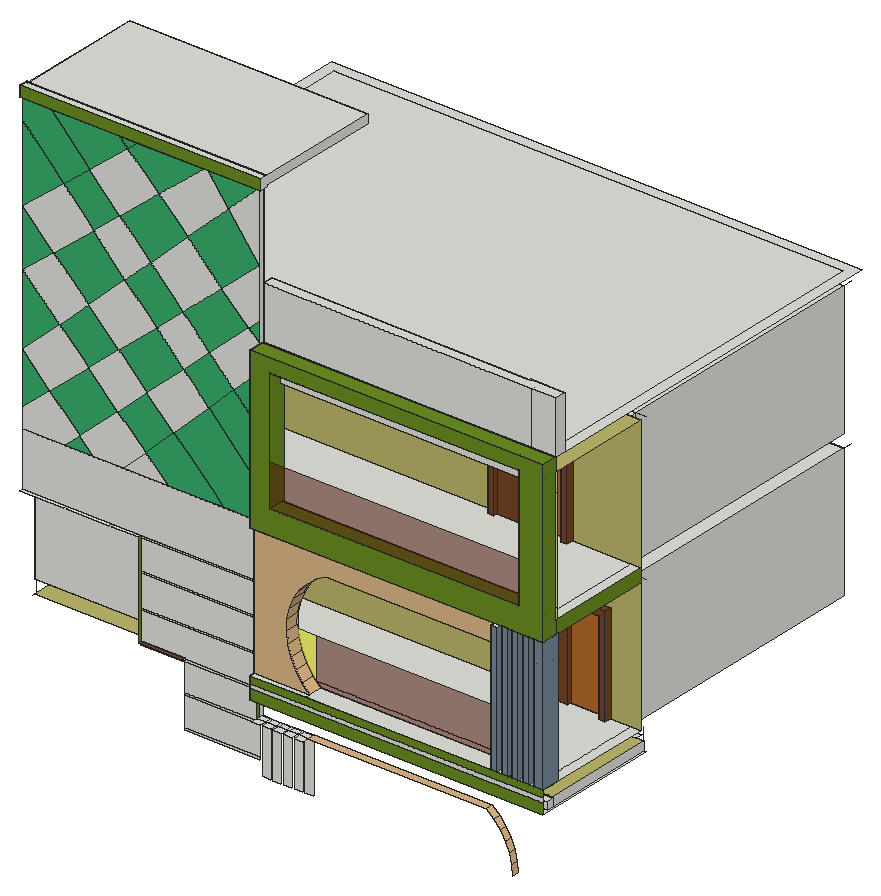
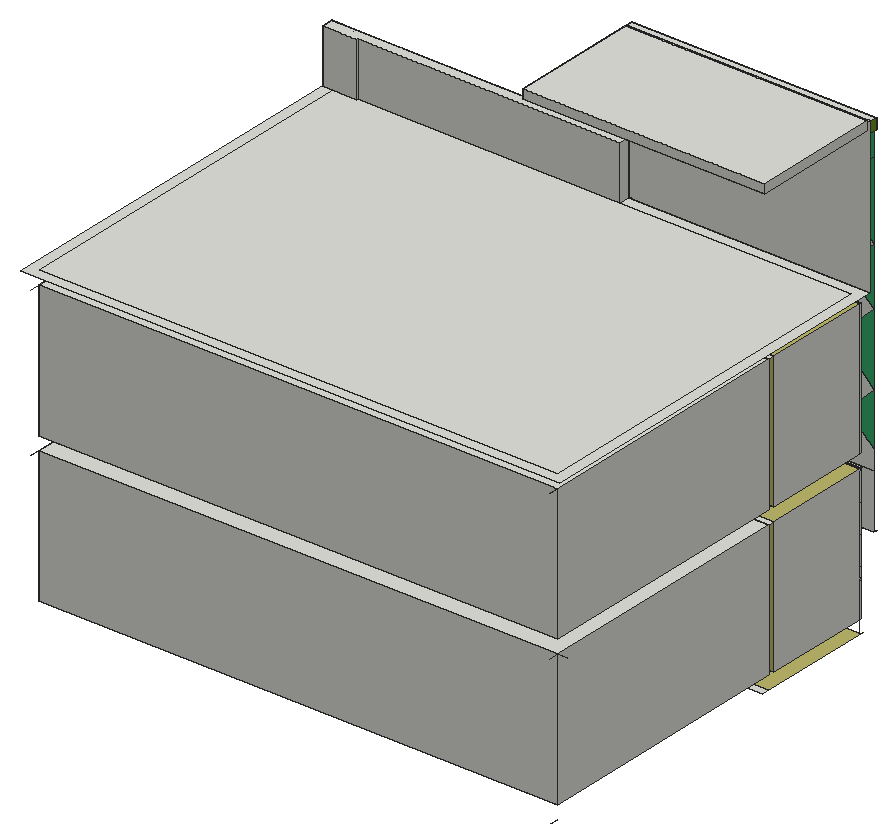
# SketchUp Ruby script. Lengths in inches.
U = 1.inch
M = Sketchup.active_model
def pt(a) = Geom::Point3d.new(a.map { |v| v * U })
def face(e, loops, mat)
  f = e.add_face(loops[0].map { |a| pt(a) })
  loops[1..].each { |l| e.add_face(l.map { |a| pt(a) }).erase! }
  f.material = f.back_material = mat if mat
  f
end
# faces: each face lists its corners as indices into pts; further lists are holes
def faces(e, pts, list, mat = nil) = list.each { |f| face(e, (f[0].is_a?(Array) ? f : [f]).map { |l| l.map { |i| pts[i] } }, mat) }
# xy, xz, yz: faces in a plane at the given z, y or x. An outline is a flat list of corners, or four numbers for a rectangle; further outlines are holes
def ring(l) = l.size == 4 ? [[l[0], l[1]], [l[2], l[1]], [l[2], l[3]], [l[0], l[3]]] : l.each_slice(2).to_a
def flat(e, list, mat, &to3) = list.each { |f| face(e, (f[0].is_a?(Array) ? f : [f]).map { |l| ring(l).map { |u, v| to3.(u, v) } }, mat) }
def xy(e, z, list, mat = nil) = flat(e, list, mat) { |x, y| [x, y, z] }
def xz(e, y, list, mat = nil) = flat(e, list, mat) { |x, z| [x, y, z] }
def yz(e, x, list, mat = nil) = flat(e, list, mat) { |y, z| [x, y, z] }
def lines(e, pts, list) = list.each { |a, b| e.add_line(pt(pts[a]), pt(pts[b])) }
# prism: a flat outline (further loops are holes) pulled along v
def prism(e, loops, v, mat = nil)
  f = face(e, loops, mat); d = Geom::Vector3d.new(v.map { |x| x * U })
  f.pushpull(f.normal.samedirection?(d) ? d.length : -d.length)
end
def box(e, o, s, mat = nil) = prism(e, [[o, [o[0] + s[0], o[1], o[2]], [o[0] + s[0], o[1] + s[1], o[2]], [o[0], o[1] + s[1], o[2]]]], [0, 0, s[2]], mat)
def at(x, y, z, deg = 0) = Geom::Transformation.translation(pt([x, y, z])) * Geom::Transformation.rotation(ORIGIN, Z_AXIS, deg.degrees)
def axes(o, x, y, z) = Geom::Transformation.new([*x, 0, *y, 0, *z, 0, *pt(o).to_a, 1])
def part(name) = M.definitions.add(name)
# library, detail: a bought-in or finely detailed component or shape, given as its bounding box
def library(name, o, s) = part(name).tap { |d| box(d.entities, o, s) }
def detail(e, o, s) = box(e.add_group.entities, o, s)
def put(e, d, t, mat = nil) = e.add_instance(d, t).tap { |i| i.material = mat if mat }
def group(e, t, mat = nil) = e.add_group.tap { |g| g.transformation = t; g.material = mat if mat }.entities
root = M.entities
M.materials.add("[0036_BurlyWood]").color = [222, 184, 135]
M.materials.add("[0057_DarkKhaki]").color = [189, 183, 107]
M.materials.add("[0061_OliveDrab]").color = [107, 142, 35]
M.materials.add("[0074_SeaGreen]").color = [57, 173, 108]
M.materials.add("[0110_LightSlateGray]").color = [119, 136, 153]
M.materials.add("[Sandstone]").color = [118, 81, 52]
M.materials.add("[Translucent Glass Dark Green]").color = [91, 24, 11]
M.materials["[Translucent Glass Dark Green]"].alpha = 0.5
M.materials.add("[Translucent Glass Gold]").color = [255, 254, 26]
M.materials["[Translucent Glass Gold]"].alpha = 0.6
M.materials.add("[Translucent Glass Gray]").color = [128, 128, 128]
M.materials["[Translucent Glass Gray]"].alpha = 0.5
M.materials.add("[Wood Bamboo]").color = [177, 105, 43]
M.materials.add("[Wood Cherry Original]").color = [152, 86, 42]
M.materials.add("[Wood Veneer 01]").color = [120, 70, 37]
xy(root,302.01,[[383.79,177.4375,383.79,179.4375,386.62,179.4375,386.62,178.4375,395.22,178.4375,395.22,179.4375,398.06,179.4375,398.06,177.4375]],"[Wood Veneer 01]")
xy(root,303.76,[[383.79,177.4375,398.06,177.4375,398.06,179.4375,395.22,179.4375,395.22,178.4375,386.62,178.4375,386.62,179.4375,383.79,179.4375]],"[Wood Veneer 01]")
xy(root,336,[[379.35,179.4375,409.35,182.4375]])
xy(root,336,[[379.35,176.4375,409.35,179.4375],[409.35,176.4375,439.35,182.4375]],"[Wood Veneer 01]")
xy(root,338.33,[[301.39,179.4375,326.48,182.4375],[329.2,179.4375,351.57,182.4375]],"[Wood Cherry Original]")
xy(root,341.33,[[298.39,179.4375,354.57,182.4375]],"[Wood Cherry Original]")
xy(root,342,[[373.35,176.4375,445.35,182.4375]],"[Wood Veneer 01]")
xy(root,345.55,[[214.69,67.75,222.11,73.75],[224.38,67.75,231.79,73.75],[234.07,67.75,241.48,73.75],[243.75,67.75,251.17,73.75],[253.44,67.75,260.86,73.75],
  [214.69,73.75,222.11,79.75],[222.11,73.75,224.38,79.75],[224.38,73.75,231.79,79.75],[231.79,73.75,234.07,79.75],[234.07,73.75,241.48,79.75],
  [241.48,73.75,243.75,79.75],[243.75,73.75,251.17,79.75],[251.17,73.75,253.44,79.75],[253.44,73.75,260.86,79.75]])
xy(root,345.55,[[260.86,73.75,422.69,79.75]],"[0036_BurlyWood]")
xy(root,363.8125,[[214.69,65.75,214.69,73.75,477.8125,73.75,477.8125,182.4375,480,182.4375,480,65.75]])
xy(root,369.44,[[107.35,73.75,146.78,76.75]],"[Sandstone]")
xy(root,370.625,[[214.69,73.75,477.8125,79.75,477.8125,73.75]])
xy(root,372,[[9,182.4375,471,188.4375]])
xy(root,372,[[9,79.75,477.8125,182.4375]],"[0057_DarkKhaki]")
xy(root,384,[[214.69,65.75,264.77,70.3125],[264.77,65.75,432.6,82.75],[432.6,65.75,438.3,82.75],[438.3,65.75,442.22,82.75],[442.22,65.75,447.93,82.75],
  [447.93,65.75,451.85,82.75],[451.85,65.75,457.55,82.75],[457.55,65.75,461.47,82.75],[461.47,65.75,467.18,82.75],[467.18,65.75,471.78,82.75],
  [471.78,65.75,480,76.75],[214.69,70.3125,264.77,76.75],[214.69,76.75,264.77,79.75],[471.78,76.75,480,77.8125],[471.78,77.8125,480,82.75],
  [9,79.75,214.69,81.3125],[214.69,79.75,264.77,79.75,264.77,82.75,244.77,82.75,244.77,82.4375,214.69,82.4375],[9,81.3125,214.69,81.3125,214.69,82.75,480,82.75,480,176.4375,471,176.4375,471,88.75,9,88.75],[214.69,82.4375,244.77,82.75],[9,88.75,471,88.75,471,176.4375,452.43,176.4375,452.43,170.4375,446.43,170.4375,446.43,176.4375,416.43,176.4375,416.43,173.4375,386.43,173.4375,386.43,170.4375,380.43,170.4375,380.43,176.4375,9,176.4375],
  [380.43,170.4375,386.43,176.4375],[446.43,170.4375,452.43,176.4375],[386.43,173.4375,416.43,176.4375],[9,182.4375,471,417.3125]])
xy(root,415.43,[[290.01,173.4375,348.2,176.4375]])
xy(root,418.43,[[293.01,173.4375,319.1,176.4375],[322.56,173.4375,345.2,176.4375]],"[Wood Cherry Original]")
xy(root,433.625,[[389.68,170.4375,390.18,171.4375],[389.68,171.4375,390.18,173.4375]],"[Wood Veneer 01]")
xy(root,434.43,[[389.68,171.4375,390.18,173.4375]],"[Wood Veneer 01]")
xy(root,440.6875,[[389.68,171.4375,390.18,173.4375]],"[Wood Veneer 01]")
xy(root,441.5,[[389.68,170.4375,390.18,171.4375],[389.68,171.4375,390.18,173.4375]],"[Wood Veneer 01]")
xy(root,455,[[0,73.75,39.7,76.75],[42.34,73.75,80.57,76.75],[83.22,73.75,107.35,76.75]])
xy(root,468,[[386.43,173.4375,416.43,176.4375]])
xy(root,468,[[386.43,170.4375,416.43,173.4375],[416.43,170.4375,446.43,176.4375]],"[Wood Veneer 01]")
xy(root,474,[[380.43,170.4375,452.43,176.4375]],"[Wood Veneer 01]")
xy(root,478.24,[[293.01,173.4375,319.1,176.4375],[322.56,173.4375,345.2,176.4375]],"[Wood Cherry Original]")
xy(root,481.24,[[290.01,173.4375,348.2,176.4375]])
xy(root,484.84,[[279.79,82.4375,471.78,82.75]])
xy(root,484.84,[[279.79,70.3125,471.78,76.75]],"[0036_BurlyWood]")
xy(root,501.3125,[[432.6,65.75,438.3,82.75]])
xy(root,504,[[214.69,65.75,442.22,67.21],[442.22,65.75,447.93,70.3125],[447.93,65.75,451.85,67.21],[451.85,65.75,457.55,67.21],[457.55,65.75,461.47,67.21],
  [461.47,65.75,467.18,67.21],[467.18,65.75,471.78,67.21],[471.78,65.75,473.53,67.21],[473.53,65.75,480,67.21],[214.69,67.21,442.22,70.3125],
  [447.93,67.21,451.85,70.3125],[451.85,67.21,457.55,70.3125],[457.55,67.21,461.47,70.3125],[461.47,67.21,467.18,70.3125],[467.18,67.21,471.78,70.3125],
  [471.78,67.21,473.53,70.3125],[473.53,67.21,480,76.75],[214.69,70.3125,442.22,76.75],[442.22,70.3125,447.93,76.75],[447.93,70.3125,451.85,76.75],
  [451.85,70.3125,457.55,76.75],[457.55,70.3125,461.47,76.75],[461.47,70.3125,467.18,76.75],[467.18,70.3125,471.78,76.75],[471.78,70.3125,473.53,76.75],
  [9,76.75,214.69,79.75],[214.69,76.75,442.22,79.75],[442.22,76.75,447.93,79.75],[447.93,76.75,451.85,79.75],[451.85,76.75,457.55,79.75],
  [457.55,76.75,461.47,79.75],[461.47,76.75,467.18,79.75],[467.18,76.75,471.78,79.75],[471.78,76.75,473.53,79.75],[473.53,76.75,480,79.75],
  [9,79.75,214.69,81.3125],[214.69,79.75,451.85,82.4375],[451.85,79.75,457.55,82.4375],[457.55,79.75,461.47,82.4375],[461.47,79.75,467.18,82.4375],
  [467.18,79.75,471.78,82.4375],[471.78,79.75,480,82.75],[214.69,82.4375,451.85,82.75],[451.85,82.4375,457.55,82.75],[457.55,82.4375,461.47,82.75],
  [461.47,82.4375,467.18,82.75],[467.18,82.4375,471.78,82.75],[9,176.4375,471,182.4375],[9,182.4375,471,417.3125]])
xy(root,504,[[9,81.3125,9,176.4375,480,176.4375,480,82.75,214.69,82.75,214.69,81.3125]],"[0057_DarkKhaki]")
xy(root,504.25,[[442.22,65.75,447.93,67.21],[442.22,67.21,447.93,79.75],[442.22,79.75,447.93,82.75]])
xy(root,516,[[232.86,79.75,471,79.75,471,176.4375,418.0625,176.4375,418.0625,170.4375,412.0625,170.4375,412.0625,176.4375,382.0625,176.4375,382.0625,173.4375,352.0625,173.4375,352.0625,170.4375,346.0625,170.4375,346.0625,176.4375,9,176.4375,9,81.3125,214.69,81.3125,214.69,81.21,232.86,81.21],[9,79.75,214.69,81.3125],[214.69,79.75,232.86,81.21],[471,79.75,480,176.4375],[346.0625,170.4375,352.0625,176.4375],
  [412.0625,170.4375,418.0625,176.4375],[352.0625,173.4375,382.0625,176.4375],[9,182.4375,471,417.3125]])
xy(root,525.77,[[232.86,65.75,458.23,79.75]],"[0061_OliveDrab]")
xy(root,557.24,[[255.7,173.4375,311.2,176.4375]])
xy(root,560.24,[[258.7,173.4375,283.45,176.4375],[285.78,173.4375,308.2,176.4375]],"[Wood Cherry Original]")
xy(root,560.85,[[354.3,171.4375,355.24,173.4375]])
xy(root,563.35,[[354.3,172.4375,355.24,173.4375]],"[Wood Veneer 01]")
xy(root,570.73,[[354.3,172.4375,355.24,173.4375]])
xy(root,573.23,[[354.3,171.4375,355.24,173.4375]],"[Wood Veneer 01]")
xy(root,600,[[352.0625,170.4375,382.0625,173.4375],[382.0625,170.4375,412.0625,176.4375]],"[Wood Veneer 01]")
xy(root,606,[[346.0625,170.4375,418.0625,176.4375]],"[Wood Veneer 01]")
xy(root,609.74,[[258.7,173.4375,283.45,176.4375],[285.78,173.4375,308.2,176.4375]],"[Wood Cherry Original]")
xy(root,612.74,[[255.7,173.4375,311.2,176.4375]],"[Wood Cherry Original]")
xy(root,622.99,[[458.2,75.25,232.83,76.58,232.86,81.21,458.23,79.88,458.23,79.75]])
xy(root,636,[[458.2,75.25,232.86,76.58,232.86,79.75,458.23,79.75],[232.83,76.58,232.86,76.58,232.86,79.75,232.85,79.75],[9,79.75,214.69,81.3125],[214.69,79.75,232.85,79.75,232.86,81.21,214.69,81.21],[232.86,79.75,232.86,81.21,214.69,81.21,214.69,81.3125,232.86,81.21,458.23,79.88,458.23,79.75],
  [232.85,79.75,232.86,79.75,232.86,81.21],[9,176.4375,471,182.4375],[9,182.4375,471,417.3125]])
xy(root,636,[[480,79.75,458.23,79.88,232.86,81.21,214.69,81.3125,9,81.3125,9,176.4375,480,176.4375]],"[0057_DarkKhaki]")
xy(root,636,[[232.86,65.75,458.23,67.21],[232.86,67.21,232.86,76.58,458.2,75.25,458.23,79.75,458.23,67.21]],"[0061_OliveDrab]")
xy(root,648,[[214.69,79.75,458.23,79.75,458.23,79.88,214.69,81.3125],[458.23,79.75,480,79.75,458.23,79.88],[480,79.75,480,79.88,458.23,79.88],[458.23,79.88,214.69,81.3125,214.72,90.3125,449.23,88.93,449.23,90.21,480,90.21,480,82.71,458.23,82.71],[458.23,79.88,480,80.14],
  [458.23,80.14,480,81.21],[458.23,81.21,480,82.71],[0,81.3125,214.69,81.3125,214.72,90.3125,9,90.3125,9,417.3125,471,417.3125,471,90.21,480,90.21,480,426.3125,0,426.3125],[449.23,88.93,449.23,90.21,471,90.21,471,417.3125,9,417.3125,9,90.3125,214.72,90.3125]])
xy(root,648,[[214.69,65.75,480,79.75]],"[0061_OliveDrab]")
xy(root,696,[[458.23,79.88,480,79.88,480,90.21,449.23,90.21,449.23,88.93,214.72,90.3125,214.69,81.3125]])
xy(root,774.38,[[0,76.75,22.45,79.75],[22.45,76.75,85.57,79.75],[85.57,76.75,107.35,79.75],[107.35,76.75,166.47,79.75],[166.47,76.75,214.69,79.75]])
xy(root,774.38,[[0,73.75,22.45,76.75],[22.45,73.75,85.57,76.75],[85.57,73.75,107.35,76.75],[107.35,73.75,166.47,76.75],[166.47,73.75,166.47,76.75,214.69,76.75,214.69,81.3125,217.75,81.3125,217.75,73.75]],"[0061_OliveDrab]")
xy(root,775.875,[[2.13,81.3125,217.75,194.875]])
xy(root,784.0625,[[0,73.75,217.75,79.75],[0,79.75,2.13,81.3125],[2.13,79.75,217.75,81.3125],[2.13,81.3125,217.75,194.875]])
xz(root,65.75,[[214.69,373.91,480,377.57],[442.22,504,447.93,504.25]])
xz(root,65.75,[[214.69,363.8125,480,373.91],[214.69,377.57,480,384],[[214.69,504,442.22,504,442.22,504.25,447.93,504.25,447.93,504,480,504,480,648,214.69,648],[232.86,525.77,458.23,636]]],"[0061_OliveDrab]")
xz(root,65.75,[[432.6,384,438.3,501.3125],[442.22,384,447.93,504],[451.85,384,457.55,504],[461.47,384,467.18,504],[471.78,384,480,504]],"[0110_LightSlateGray]")
xz(root,65.75,[[232.86,525.77,458.23,563.72]],"[Translucent Glass Dark Green]")
xz(root,70.3125,[[471.78,484.84,473.53,504]])
xz(root,70.3125,[[214.69,384,264.77,384,257.77,391.25,252.07,399.57,247.82,408.71,245.15,418.43,244.12,428.46,244.77,438.52,247.08,448.33,250.99,457.625,256.375,466.14,263.1,473.65,270.98,479.94,279.79,484.84,471.78,484.84,471.78,504,214.69,504]],"[0036_BurlyWood]")
xz(root,73.75,[[214.69,363.8125,477.8125,370.625]])
xz(root,73.75,[[0,774.38,217.75,784.0625]],"[0061_OliveDrab]")
xz(root,76.75,[[146.78,310.89,214.69,312.74],[146.78,312.74,214.69,339.34],[146.78,339.34,214.69,341.2],[146.78,341.2,214.69,341.2,214.69,366.59,107.35,366.59,107.35,369.44,146.78,369.44],[107.35,366.59,146.78,368.45],
  [146.78,366.59,214.69,368.45],[107.35,368.45,146.78,369.44],[146.78,368.45,214.69,368.45,214.69,394.84,107.35,394.84,107.35,369.44,146.78,369.44],[107.35,394.84,214.69,396.7],[107.35,396.7,214.69,424.34],
  [107.35,424.34,214.69,426.2],[107.35,426.2,214.69,453.13],[107.35,453.13,214.69,455],[0,455,214.69,504],[0,504,38.29,504,52.01,516.65,24.94,543.56,0,521.52],
  [64.73,504,91.18,504,111.25,523.71,86.25,548.21,52.01,516.65],[91.18,504,131.37,504,111.25,523.71],[24.94,543.56,59.68,574.24,33.18,600.2,0,568.36],[86.25,548.21,112.7,572.59,86.87,598.27,59.68,574.24],[136.72,548.71,168.17,579.59,145.625,602.94,112.7,572.59],
  [86.87,598.27,121.02,628.4375,92.93,657.54,59.51,625.47],[33.18,600.2,59.51,625.47,28.14,656.66,0,632.72],[191.26,602.27,214.69,625.27,214.69,647.875,204.84,657.53,169.24,624.71],[145.625,602.94,169.24,624.71,144.9,649.53,121.02,628.4375],[144.9,649.53,180.71,681.17,149.46,711.79,115.66,679.35],
  [28.14,656.66,64.18,687.33,36.96,715.53,0,684.63],[204.84,657.53,214.69,666.6,214.69,711.19,180.71,681.17],[92.93,657.54,115.66,679.35,87.97,707.58,64.18,687.33],[87.97,707.58,123.18,737.54,95.6,764.5625,60.7,735.38],[214.69,711.19,214.69,774.38,186.85,747.67],
  [149.46,711.79,186.85,747.67,166.47,774.38,123.18,737.54]])
xz(root,76.75,[[38.29,504,64.73,504,52.01,516.65],[131.37,504,181.6875,504,136.72,548.71,111.25,523.71],[181.6875,504,214.69,504,214.69,531.38,168.17,579.59,136.72,548.71],[52.01,516.65,86.25,548.21,59.68,574.24,24.94,543.56],[0,521.52,24.94,543.56,0,568.36],
  [111.25,523.71,136.72,548.71,112.7,572.59,86.25,548.21],[214.69,531.38,214.69,578.38,191.26,602.27,168.17,579.59],[0,568.36,33.18,600.2,0,632.72],[112.7,572.59,145.625,602.94,121.02,628.4375,86.87,598.27],[59.68,574.24,86.87,598.27,59.51,625.47,33.18,600.2],
  [214.69,578.38,214.69,625.27,191.26,602.27],[168.17,579.59,191.26,602.27,169.24,624.71,145.625,602.94],[169.24,624.71,204.84,657.53,180.71,681.17,144.9,649.53],[59.51,625.47,92.93,657.54,64.18,687.33,28.14,656.66],[121.02,628.4375,144.9,649.53,115.66,679.35,92.93,657.54],
  [0,632.72,28.14,656.66,0,684.63],[214.69,647.875,214.69,666.6,204.84,657.53],[115.66,679.35,149.46,711.79,123.18,737.54,87.97,707.58],[180.71,681.17,214.69,711.19,186.85,747.67,149.46,711.79],[0,684.63,36.96,715.53,0,753.83],
  [64.18,687.33,87.97,707.58,60.7,735.38,36.96,715.53],[36.96,715.53,60.7,735.38,22.45,774.38,0,774.38,0,753.83],[60.7,735.38,95.6,764.5625,85.57,774.38,22.45,774.38],[123.18,737.54,166.47,774.38,107.35,774.38,95.6,764.5625],[186.85,747.67,214.69,774.38,166.47,774.38],
  [95.6,764.5625,107.35,774.38,85.57,774.38]],"[0074_SeaGreen]")
xz(root,79.75,[[214.69,296.15,222.11,345.55],[224.38,296.15,231.79,345.55],[234.07,296.15,241.48,345.55],[243.75,296.15,251.17,345.55],[253.44,296.15,260.86,345.55],
  [214.69,370.625,477.8125,372],[9,384,214.69,504],[214.69,504,214.69,516,480,516,480,504,447.93,504,447.93,504.25,442.22,504.25,442.22,504],[442.22,504,447.93,504.25],[9,516,214.69,636],
  [232.86,516,232.86,525.77,458.23,525.77,458.23,636,214.69,636,214.69,648,480,648,480,516]])
xz(root,79.88,[[458.23,648,480,696]])
xz(root,81.21,[[214.69,516,232.86,636]])
xz(root,81.3125,[[0,647.875,214.69,648],[0,648,0,784.0625,2.13,784.0625,2.13,775.875,217.75,775.875,217.75,774.38,214.69,774.38,214.69,648]])
xz(root,82.4375,[[214.69,384,244.77,384,244.77,422.09,244.44,425.34,244.12,428.46,244.77,438.52,247.08,448.33,250.99,457.625,256.375,466.14,263.1,473.65,270.98,479.94,279.79,484.84,471.78,484.84,471.78,504,214.69,504]],"[0057_DarkKhaki]")
xz(root,82.75,[[214.69,384,214.69,504,442.22,504,442.22,484.84,438.3,484.84,438.3,501.3125,432.6,501.3125,432.6,484.84,279.79,484.84,270.98,479.94,263.1,473.65,256.375,466.14,250.99,457.625,247.08,448.33,244.77,438.52,244.12,428.46,244.44,425.34,244.77,422.09,244.77,384],[244.77,384,244.77,422.09,245.15,418.43,247.82,408.71,252.07,399.57,257.77,391.25,264.77,384],[432.6,384,438.3,425.34],[438.3,384,442.22,425.34],[442.22,384,447.93,425.34],
  [447.93,384,451.85,425.34],[451.85,384,457.55,425.34],[457.55,384,461.47,425.34],[461.47,384,467.18,425.34],[467.18,384,471.78,425.34],
  [471.78,384,480,504],[244.77,422.09,244.44,425.34,244.77,425.34],[244.44,425.34,244.12,428.46,244.77,438.52,244.77,425.34],[432.6,425.34,438.3,484.84],[442.22,425.34,447.93,484.84],
  [451.85,425.34,457.55,484.84],[461.47,425.34,467.18,484.84],[432.6,484.84,438.3,501.3125],[442.22,484.84,447.93,504],[447.93,484.84,451.85,504],
  [451.85,484.84,457.55,504],[457.55,484.84,461.47,504],[461.47,484.84,467.18,504],[467.18,484.84,471.78,504],[442.22,504,447.93,504.25]])
xz(root,82.75,[[264.77,384,432.6,384,432.6,425.34,261.27,425.34,261.27,387.625]],"[Translucent Glass Dark Green]")
xz(root,82.75,[[261.27,387.625,257.77,391.25,252.07,399.57,247.82,408.71,245.15,418.43,244.77,422.09,244.77,425.34,261.27,425.34]],"[Translucent Glass Gold]")
xz(root,90.21,[[449.23,648,480,696]])
xz(root,170.4375,[[380.43,384,386.43,384,386.43,468,446.43,468,446.43,384,452.43,384,452.43,474,380.43,474],[389.68,433.625,390.18,441.5],[346.0625,516,352.0625,516,352.0625,600,412.0625,600,412.0625,516,418.0625,516,418.0625,606,346.0625,606]],"[Wood Veneer 01]")
xz(root,171.4375,[[389.68,434.43,390.18,440.6875]])
xz(root,171.4375,[[354.3,560.85,355.24,573.23]],"[Wood Veneer 01]")
xz(root,172.4375,[[354.3,563.35,355.24,570.73]])
xz(root,173.4375,[[[290.01,415.43,348.2,481.24],[293.01,418.43,319.1,478.24],[322.56,418.43,345.2,478.24]],[[255.7,557.24,311.2,612.74],[258.7,560.24,283.45,609.74],[285.78,560.24,308.2,609.74]]],"[Wood Cherry Original]")
xz(root,173.4375,[[[386.43,384,416.43,468],[389.68,440.6875,390.18,441.5],[389.68,433.625,390.18,434.43]],[[352.0625,516,382.0625,600],[354.3,570.73,355.24,573.23],[354.3,560.85,355.24,563.35]]],"[Wood Veneer 01]")
xz(root,176.4375,[[380.43,378,452.43,384],[380.43,384,380.43,474,452.43,474,452.43,384,446.43,384,446.43,468,386.43,468,386.43,384],[[290.01,415.43,348.2,481.24],[293.01,418.43,319.1,478.24],[322.56,418.43,345.2,478.24]],[471,504,480,516],[346.0625,510,418.0625,516],
  [[255.7,557.24,311.2,612.74],[258.7,560.24,283.45,609.74],[285.78,560.24,308.2,609.74]]])
xz(root,176.4375,[[[9,384,380.43,384,380.43,474,452.43,474,452.43,384,480,384,480,504,9,504],[290.01,415.43,348.2,481.24]],[[9,516,346.0625,516,346.0625,606,418.0625,606,418.0625,516,480,516,480,636,9,636],[255.7,557.24,311.2,612.74]]],"[0057_DarkKhaki]")
xz(root,176.4375,[[293.01,418.43,319.1,478.24],[322.56,418.43,345.2,478.24],[258.7,560.24,283.45,609.74],[285.78,560.24,308.2,609.74]],"[Translucent Glass Gray]")
xz(root,176.4375,[[416.43,384,446.43,468],[382.0625,516,412.0625,600]],"[Wood Bamboo]")
xz(root,177.4375,[[383.79,302.01,398.06,303.76]],"[Wood Veneer 01]")
xz(root,178.4375,[[386.62,302.01,395.22,303.76]])
xz(root,179.4375,[[383.79,302.01,386.62,303.76],[395.22,302.01,398.06,303.76]])
xz(root,182.4375,[[9,384,471,504],[9,516,471,636]])
xz(root,194.875,[[2.13,775.875,217.75,784.0625]])
xz(root,417.3125,[[9,384,471,504],[9,516,471,636]])
yz(root,0,[[73.75,774.38,79.75,784.0625]],"[0061_OliveDrab]")
yz(root,2.13,[[81.3125,775.875,194.875,784.0625]])
yz(root,9,[[79.75,384,81.3125,504],[81.3125,384,176.4375,504],[182.4375,384,417.3125,504],[79.75,516,81.3125,636],[81.3125,516,176.4375,636],
  [182.4375,516,417.3125,636]])
yz(root,107.35,[[73.75,369.44,76.75,455]],"[0061_OliveDrab]")
yz(root,214.69,[[76.75,345.55,79.75,345.55,79.75,370.625,76.75,367.4375],[76.75,367.4375,79.75,370.625,79.75,384,76.75,384],[70.3125,384,76.75,504],[76.75,384,79.75,504],[79.75,384,82.4375,504],
  [82.4375,384,82.75,504],[76.75,504,79.75,516],[79.75,504,81.21,516],[81.21,504,81.3125,516],[76.75,516,79.75,636],
  [79.75,516,81.21,526.5],[79.75,526.5,81.21,636],[76.75,636,79.75,647.875],[79.75,636,81.3125,647.875],[76.75,647.875,79.75,648],
  [79.75,647.875,81.3125,648],[76.75,648,79.75,774.38],[79.75,648,81.3125,774.38]])
yz(root,214.69,[[73.75,345.55,73.75,370.625,76.75,367.4375,76.75,345.55],[65.75,363.8125,65.75,384,76.75,384,76.75,367.4375,73.75,370.625,73.75,363.8125],[65.75,504,67.21,648],[67.21,504,76.75,648]],"[0061_OliveDrab]")
yz(root,217.75,[[73.75,774.38,81.3125,774.38,81.3125,775.875,194.875,775.875,194.875,784.0625,73.75,784.0625]])
yz(root,232.86,[[79.75,516,81.21,516,81.21,636,65.75,636,65.75,525.77,79.75,525.77]],"[0061_OliveDrab]")
yz(root,244.77,[[82.4375,384,82.75,422.09]])
yz(root,255.7,[[173.4375,557.24,176.4375,612.74]])
yz(root,258.7,[[173.4375,560.24,176.4375,609.74]],"[Wood Cherry Original]")
yz(root,283.45,[[173.4375,560.24,176.4375,609.74]])
yz(root,285.78,[[173.4375,560.24,176.4375,609.74]],"[Wood Cherry Original]")
yz(root,290.01,[[173.4375,415.43,176.4375,481.24]])
yz(root,293.01,[[173.4375,418.43,176.4375,478.24]],"[Wood Cherry Original]")
yz(root,308.2,[[173.4375,560.24,176.4375,609.74]],"[Wood Cherry Original]")
yz(root,311.2,[[173.4375,557.24,176.4375,612.74]],"[Wood Cherry Original]")
yz(root,319.1,[[173.4375,418.43,176.4375,478.24]],"[Wood Cherry Original]")
yz(root,322.56,[[173.4375,418.43,176.4375,478.24]],"[Wood Cherry Original]")
yz(root,345.2,[[173.4375,418.43,176.4375,478.24]],"[Wood Cherry Original]")
yz(root,346.0625,[[170.4375,516,176.4375,606]],"[Wood Veneer 01]")
yz(root,348.2,[[173.4375,415.43,176.4375,481.24]],"[Wood Cherry Original]")
yz(root,352.0625,[[170.4375,516,173.4375,600]],"[Wood Veneer 01]")
yz(root,354.3,[[171.4375,560.85,171.4375,573.23,173.4375,573.23,173.4375,570.73,172.4375,570.73,172.4375,563.35,173.4375,563.35,173.4375,560.85]],"[Wood Veneer 01]")
yz(root,355.24,[[171.4375,560.85,173.4375,560.85,173.4375,563.35,172.4375,563.35,172.4375,570.73,173.4375,570.73,173.4375,573.23,171.4375,573.23]],"[Wood Veneer 01]")
yz(root,380.43,[[170.4375,384,176.4375,474]],"[Wood Veneer 01]")
yz(root,382.0625,[[173.4375,516,176.4375,600]],"[Wood Veneer 01]")
yz(root,383.79,[[177.4375,302.01,179.4375,303.76]])
yz(root,386.43,[[173.4375,384,176.4375,468]])
yz(root,386.43,[[170.4375,384,173.4375,468]],"[Wood Veneer 01]")
yz(root,386.62,[[178.4375,302.01,179.4375,303.76]],"[Wood Veneer 01]")
yz(root,389.68,[[170.4375,433.625,170.4375,441.5,173.4375,441.5,173.4375,440.6875,171.4375,440.6875,171.4375,434.43,173.4375,434.43,173.4375,433.625]],"[Wood Veneer 01]")
yz(root,390.18,[[170.4375,433.625,173.4375,433.625,173.4375,434.43,171.4375,434.43,171.4375,440.6875,173.4375,440.6875,173.4375,441.5,170.4375,441.5]],"[Wood Veneer 01]")
yz(root,395.22,[[178.4375,302.01,179.4375,303.76]],"[Wood Veneer 01]")
yz(root,398.06,[[177.4375,302.01,179.4375,303.76]],"[Wood Veneer 01]")
yz(root,412.0625,[[170.4375,516,176.4375,600]],"[Wood Veneer 01]")
yz(root,416.43,[[173.4375,384,176.4375,468]],"[Wood Veneer 01]")
yz(root,418.0625,[[170.4375,516,176.4375,606]],"[Wood Veneer 01]")
yz(root,432.6,[[65.75,384,82.75,501.3125]],"[0110_LightSlateGray]")
yz(root,438.3,[[65.75,384,82.75,501.3125]],"[0110_LightSlateGray]")
yz(root,442.22,[[65.75,504,67.21,504.25],[67.21,504,79.75,504.25]])
yz(root,442.22,[[65.75,384,65.75,504,79.75,504,79.75,504.25,82.75,504.25,82.75,384]],"[0110_LightSlateGray]")
yz(root,446.43,[[170.4375,384,176.4375,468]],"[Wood Veneer 01]")
yz(root,447.93,[[65.75,504,67.21,504.25],[67.21,504,79.75,504.25]])
yz(root,447.93,[[65.75,384,82.75,384,82.75,504.25,79.75,504.25,79.75,504,65.75,504]],"[0110_LightSlateGray]")
yz(root,449.23,[[88.93,648,90.21,696]])
yz(root,451.85,[[65.75,384,82.75,504]],"[0110_LightSlateGray]")
yz(root,452.43,[[170.4375,384,176.4375,474]],"[Wood Veneer 01]")
yz(root,457.55,[[65.75,384,82.75,504]],"[0110_LightSlateGray]")
yz(root,458.23,[[65.75,525.77,67.21,636],[79.75,622.99,79.88,628.49],[79.75,622.99,79.88,636],[79.75,628.49,79.88,633.49],[79.75,633.49,79.88,636]])
yz(root,458.23,[[67.21,525.77,79.75,636]],"[0061_OliveDrab]")
yz(root,461.47,[[65.75,384,82.75,504]],"[0110_LightSlateGray]")
yz(root,467.18,[[65.75,384,82.75,504]],"[0110_LightSlateGray]")
yz(root,471,[[182.4375,384,417.3125,504],[182.4375,516,417.3125,636]])
yz(root,471.78,[[77.8125,384,82.75,425.34],[77.8125,425.34,82.75,484.84],[70.3125,484.84,76.75,504],[82.4375,484.84,82.75,504]])
yz(root,471.78,[[65.75,384,65.75,504,70.3125,504,70.3125,484.84,76.75,484.84,76.75,504,82.4375,504,82.4375,484.84,77.8125,484.84,77.8125,384]],"[0110_LightSlateGray]")
yz(root,477.8125,[[73.75,363.8125,79.75,370.625],[79.75,363.8125,182.4375,372]])
yz(root,480,[[79.75,516,81.21,636],[79.88,648,90.21,696]])
yz(root,480,[[65.75,504,79.75,648],[79.75,504,176.4375,516]],"[0061_OliveDrab]")
yz(root,480,[[65.75,384,82.75,504]],"[0110_LightSlateGray]")
p = [[445.37,79.75,307.78],[446.07,79.75,298.78],[446.07,73.75,298.78],[445.37,73.75,307.78],[443.3,79.75,316.56],[443.3,73.75,316.56],
  [439.9,79.75,324.92],[439.9,73.75,324.92],[435.25,79.75,332.66],[435.25,73.75,332.66],[429.47,79.75,339.59],[429.47,73.75,339.59],
  [422.69,79.75,345.55],[422.69,73.75,345.55],[214.69,73.75,370.625],[214.69,76.75,367.4375],[477.8125,79.75,370.625],[214.69,79.75,370.625],
  [257.77,82.75,391.25],[257.77,70.3125,391.25],[264.77,70.3125,384],[264.77,76.75,384],[264.77,79.75,384],[264.77,82.75,384],
  [261.27,82.75,387.625],[252.07,82.75,399.57],[252.07,70.3125,399.57],[247.82,82.75,408.71],[247.82,70.3125,408.71],[245.15,82.75,418.43],
  [245.15,70.3125,418.43],[244.77,82.75,422.09],[244.77,82.4375,422.09],[244.44,82.4375,425.34],[244.12,82.4375,428.46],[244.12,70.3125,428.46],
  [244.44,82.75,425.34],[244.12,82.75,428.46],[244.77,82.4375,438.52],[244.77,70.3125,438.52],[244.77,82.75,438.52],[247.08,82.4375,448.33],
  [247.08,70.3125,448.33],[247.08,82.75,448.33],[250.99,82.4375,457.625],[250.99,70.3125,457.625],[250.99,82.75,457.625],[256.375,82.4375,466.14],
  [256.375,70.3125,466.14],[256.375,82.75,466.14],[263.1,82.4375,473.65],[263.1,70.3125,473.65],[263.1,82.75,473.65],[270.98,82.4375,479.94],
  [270.98,70.3125,479.94],[270.98,82.75,479.94],[279.79,82.4375,484.84],[279.79,76.75,484.84],[279.79,70.3125,484.84],[279.79,82.75,484.84],
  [232.83,76.58,633.49],[232.83,76.58,628.49],[232.83,76.58,622.99],[458.2,75.25,622.99],[458.2,75.25,628.49],[458.2,75.25,633.49],
  [458.2,75.25,636],[232.86,76.58,636],[232.83,76.58,636],[458.23,79.75,622.99],[458.23,79.75,628.49],[232.86,81.21,628.49],
  [232.86,81.21,622.99],[458.23,79.88,633.49],[458.23,79.88,628.49],[458.23,79.88,622.99],[232.86,81.21,633.49],[232.86,81.21,636],
  [458.23,79.88,636],[458.23,79.75,633.49],[458.23,79.75,636],[232.85,79.75,636],[214.69,81.3125,648],[458.23,79.88,648],
  [458.23,79.88,696],[214.69,81.3125,696],[214.72,90.3125,648],[214.72,90.3125,696],[449.23,88.93,648],[449.23,88.93,696],
  [9,81.125,372],[9,81.125,384],[477.8125,182.4375,372],[477.8125,182.4375,384],[9,417.3125,372],[9,426.3125,372],
  [9,417.3125,504],[9,426.3125,504],[471,417.3125,504],[471,426.3125,504],[471,182.4375,504],[480,182.4375,504],
  [0,417.3125,504],[9,417.3125,636],[9,426.3125,636],[471,417.3125,636],[471,426.3125,636],[471,182.4375,636],
  [480,182.4375,636],[214.69,81.3125,384],[214.69,81.3125,372],[9,76.75,372],[9,79.75,372],[458.23,81.21,525.77],
  [480,81.21,525.77],[458.23,67.75,525.77],[480,67.75,525.77],[458.23,81.21,648],[458.23,67.75,636],[458.23,67.75,648],
  [480,76.75,484.84],[471.78,76.75,484.84],[473.53,65.75,484.84],[473.53,70.3125,484.84],[458.23,79.75,525.77],[214.69,79.75,526.5],
  [232.86,79.75,526.5],[458.23,81.21,696],[458.23,82.71,648],[458.23,82.71,696],[480,67.75,636],[458.23,80.14,648],
  [458.23,80.14,696]]
faces(root,p,[[0,1,2,3],[4,0,3,5],[6,4,5,7],[8,6,7,9],[10,8,9,11],[12,10,11,13],[18,19,20,21,22,23,24],[25,26,19,18],
  [27,28,26,25],[29,30,28,27],[29,31,32,33,34,35,30],[38,39,35,34],[41,42,39,38],[44,45,42,41],[47,48,45,44],[50,51,48,47],
  [53,54,51,50],[56,57,58,54,53]],"[0036_BurlyWood]")
faces(root,p,[[14,15,16],[17,16,15],[36,33,32,31],[36,37,34,33],[37,40,38,34],[40,43,41,38],[43,46,44,41],[46,49,47,44],
  [49,52,50,47],[52,55,53,50],[55,59,56,53],[60,61,62,63,64,65,66,67,68],[63,69,70,64],[61,71,72,62],[73,74,75,72,71,76,77,78],[64,70,79,65],
  [60,76,71,61],[65,79,80,66],[77,76,60,68,81],[82,83,84,85],[86,82,85,87],[88,86,87,89]])
lines(root,p,[[90,91],[92,93],[94,95],[96,97],[98,99],[100,101],[96,102],[103,104],[105,106],[107,108],[109,110],[111,112],
  [113,114],[115,116],[113,117],[118,119],[120,121],[122,123],[124,113],[125,126],[117,127],[128,129],[118,130],[131,132]])
